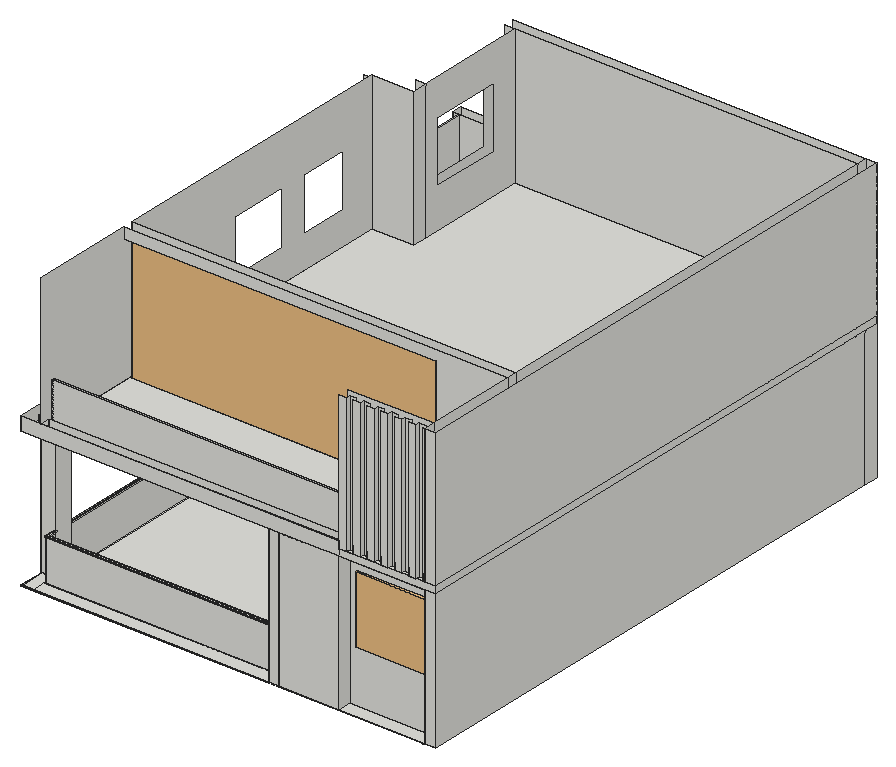
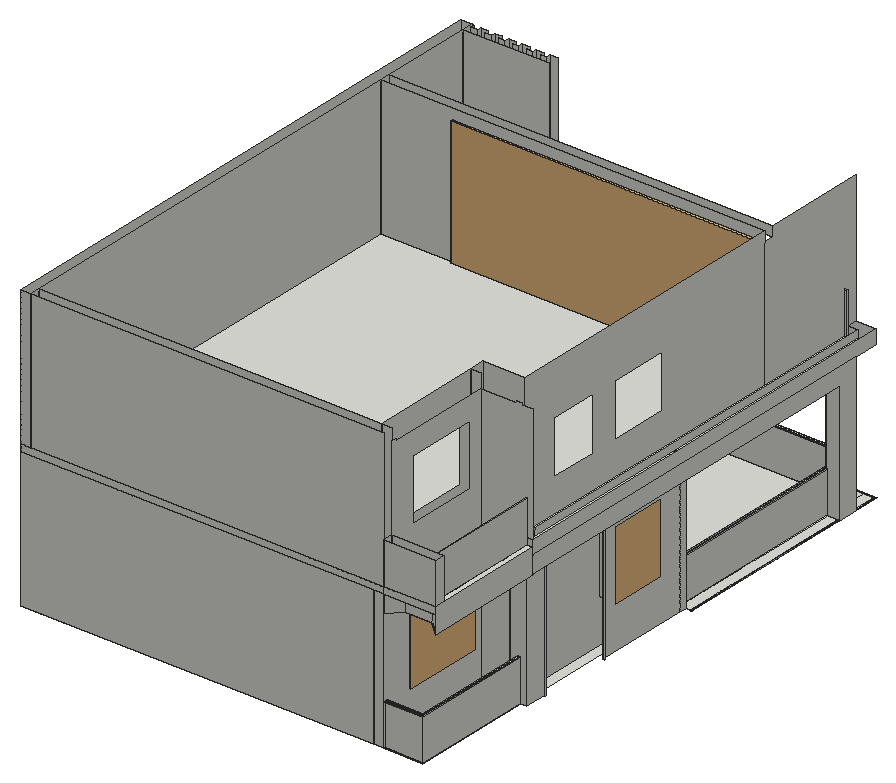
# SketchUp Ruby script. Lengths in inches.
U = 1.inch
M = Sketchup.active_model
def pt(a) = Geom::Point3d.new(a.map { |v| v * U })
def face(e, loops, mat)
  f = e.add_face(loops[0].map { |a| pt(a) })
  loops[1..].each { |l| e.add_face(l.map { |a| pt(a) }).erase! }
  f.material = f.back_material = mat if mat
  f
end
# faces: each face lists its corners as indices into pts; further lists are holes
def faces(e, pts, list, mat = nil) = list.each { |f| face(e, (f[0].is_a?(Array) ? f : [f]).map { |l| l.map { |i| pts[i] } }, mat) }
# xy, xz, yz: faces in a plane at the given z, y or x. An outline is a flat list of corners, or four numbers for a rectangle; further outlines are holes
def ring(l) = l.size == 4 ? [[l[0], l[1]], [l[2], l[1]], [l[2], l[3]], [l[0], l[3]]] : l.each_slice(2).to_a
def flat(e, list, mat, &to3) = list.each { |f| face(e, (f[0].is_a?(Array) ? f : [f]).map { |l| ring(l).map { |u, v| to3.(u, v) } }, mat) }
def xy(e, z, list, mat = nil) = flat(e, list, mat) { |x, y| [x, y, z] }
def xz(e, y, list, mat = nil) = flat(e, list, mat) { |x, z| [x, y, z] }
def yz(e, x, list, mat = nil) = flat(e, list, mat) { |y, z| [x, y, z] }
def lines(e, pts, list) = list.each { |a, b| e.add_line(pt(pts[a]), pt(pts[b])) }
# prism: a flat outline (further loops are holes) pulled along v
def prism(e, loops, v, mat = nil)
  f = face(e, loops, mat); d = Geom::Vector3d.new(v.map { |x| x * U })
  f.pushpull(f.normal.samedirection?(d) ? d.length : -d.length)
end
def box(e, o, s, mat = nil) = prism(e, [[o, [o[0] + s[0], o[1], o[2]], [o[0] + s[0], o[1] + s[1], o[2]], [o[0], o[1] + s[1], o[2]]]], [0, 0, s[2]], mat)
def at(x, y, z, deg = 0) = Geom::Transformation.translation(pt([x, y, z])) * Geom::Transformation.rotation(ORIGIN, Z_AXIS, deg.degrees)
def axes(o, x, y, z) = Geom::Transformation.new([*x, 0, *y, 0, *z, 0, *pt(o).to_a, 1])
def part(name) = M.definitions.add(name)
# library, detail: a bought-in or finely detailed component or shape, given as its bounding box
def library(name, o, s) = part(name).tap { |d| box(d.entities, o, s) }
def detail(e, o, s) = box(e.add_group.entities, o, s)
def put(e, d, t, mat = nil) = e.add_instance(d, t).tap { |i| i.material = mat if mat }
def group(e, t, mat = nil) = e.add_group.tap { |g| g.transformation = t; g.material = mat if mat }.entities
root = M.entities
c1 = library("Window 46-47",[-61.02,-2.17,0],[122.04,4.34,74.02])
c2 = library("Curtains 004",[-15.59,-2.26,0],[31.18,4.52,116.91])
c3 = library("Window 46-08",[-34.875,-3.16,0],[69.74,4.26,70.87])
c4 = library("Window 109 007",[-23.3125,-2.36,0.15],[46.625,4.71,46.28])
xy(root,383.75,[[17.25,9.625,17.25,210.85,17.3125,210.85,17.3125,9.6875,369.25,9.6875,369.25,9.625]])
xy(root,383.8125,[[17.125,9.5,17.125,210.85,17.25,210.85,17.25,9.625,369.25,9.625,369.25,9.5]])
xy(root,384,[[17.125,9.5,369.25,9.5,369.25,9.625,17.25,9.625,17.25,32.65,17.125,32.65],[17.25,9.625,369.25,9.625,369.25,9.6875,17.3125,9.6875,17.3125,32.65,17.25,32.65],[17.3125,9.6875,369.25,10.375],[17.3125,10.375,18.25,32.65],[18.25,10.375,27.25,32.65],
  [27.25,10.375,232.625,22.375],[232.625,10.375,241.625,210.85],[241.625,10.375,294.24,22.375],[294.24,10.375,369.25,22.375],[369.25,10.375,378.25,478.375],
  [27.25,22.375,232.625,22.375,232.625,23.46,28.34,23.46,28.34,32.65,27.25,32.65],[241.625,22.375,294.24,22.375,294.24,31.375,369.25,31.375,369.25,478.375,70.4375,478.375,70.4375,368.25,36.25,368.25,36.25,216.85,241.625,216.85],[294.24,22.375,369.25,31.375],[28.34,23.46,28.34,32.65,29.41,32.65,29.41,24.86,232.625,24.86,232.625,23.46],[29.41,24.86,231.54,24.86,231.54,25.95,232.625,25.95,232.625,210.85,193.58,210.85,193.58,216.85,77.58,216.85,77.58,210.85,30.5,210.85,30.5,49.65,29.41,49.65],
  [231.54,24.86,232.625,25.95],[16.4375,32.65,17.125,49.65],[17.125,32.65,17.25,49.65],[17.25,32.65,17.3125,49.65],[17.3125,32.65,29.41,49.65],
  [17.125,49.65,17.25,210.85],[17.25,49.65,17.3125,210.85],[17.3125,49.65,18.25,117.47],[18.25,49.65,27.25,210.85],[27.25,49.65,28.34,210.85],
  [28.34,49.65,29.41,210.85],[29.41,49.65,30.5,208.36],[17.3125,117.47,18.25,210.85],[29.41,208.36,30.5,209.76],[29.41,209.76,30.5,210.85],
  [22.125,210.85,27.25,216.85],[27.25,210.85,36.25,216.85],[36.25,210.85,77.58,216.85],[193.58,210.85,241.625,216.85],[27.25,216.85,36.25,384.4375],
  [36.25,368.25,70.4375,384.4375],[27.25,384.4375,28.1875,384.4375,28.1875,489.4375,61.84,489.4375,61.84,490.375,27.25,490.375],[28.1875,384.4375,28.1875,489.4375,61.84,489.4375,61.84,488.32,29.31,488.32,29.31,384.4375],[29.31,384.4375,30.25,384.4375,30.25,487.38,61.84,487.38,61.84,488.32,29.31,488.32],[30.25,384.4375,61.84,487.38],
  [61.84,384.4375,70.4375,490.375],[70.4375,478.375,378.25,490.375]])
xy(root,420,[[27.87,22.99,27.87,33.12,29.88,33.12,29.88,25.33,233.09,25.33,233.09,22.99],[27.57,23.02,27.57,30.81,27.87,31.1,27.87,23.02],[29.88,25.33,29.88,31.1,30.18,30.81,30.18,25.33],[27.79,49.1,29.96,211.4],[27.63,383.88,27.63,489.99,62.39,489.99,62.39,487.76,29.86,487.76,29.86,383.88]])
xy(root,420.5625,[[27.87,22.99,233.09,22.99,233.09,25.33,30.18,25.33,30.18,30.81,29.88,31.1,29.88,33.12,27.87,33.12,27.87,31.1,27.57,30.81,27.57,23.02,27.87,23.02],[27.63,383.88,29.86,383.88,29.86,487.76,62.39,487.76,62.39,489.99,27.63,489.99]])
xy(root,420.625,[[27.79,49.1,29.96,211.4]])
xy(root,422.29,[[22.125,240.52,36.25,287.64]])
xy(root,423.43,[[61.84,392.625,70.4375,463.11]])
xy(root,430.95,[[301.05,22.375,364.93,31.375]])
xy(root,478.55,[[61.84,392.625,70.4375,463.11]])
xy(root,479.79,[[22.125,240.52,36.25,287.64]])
xy(root,488.3125,[[16.4375,384.4375,16.4375,490.375,28.66,478.68,52.85,478.68,61.84,490.375,61.84,469.28,24.02,469.28,24.02,384.4375],[27.9,384.4375,61.84,465.4]])
xy(root,488.5,[[77.58,210.85,193.58,216.85]])
xy(root,488.88,[[16.4375,49.65,16.4375,384.4375,20.6875,384.4375,20.6875,365.41,29.41,365.41,29.41,49.65],[20.6875,365.41,22.125,384.4375]])
xy(root,489.89,[[301.05,22.375,364.93,31.375]])
xy(root,490.25,[[24.02,384.4375,24.02,469.28,61.84,469.28,61.84,465.4,27.9,465.4,27.9,384.4375]])
xy(root,504,[[[16.4375,10.375,16.4375,32.65,29.41,32.65,29.41,210.85,232.625,210.85,232.625,10.375],[52.17,29.78,206.86,176.97]],[232.625,10.375,241.625,210.85],[241.625,10.375,294.24,22.375],[294.24,10.375,369.25,22.375],[369.25,10.375,378.25,478.375],
  [241.625,22.375,241.625,216.85,70.4375,216.85,70.4375,478.375,369.25,478.375,369.25,31.375,294.24,31.375,294.24,22.375],[294.24,22.375,369.25,31.375],[294.24,22.375,369.25,31.375],[16.4375,32.65,29.41,210.85],[56.64,34.24,202.39,172.5],
  [16.4375,210.85,22.125,216.85],[22.125,210.85,29.41,216.85],[29.41,210.85,36.25,216.85],[36.25,210.85,61.84,216.85],[61.84,210.85,70.4375,216.85],
  [70.4375,210.85,241.625,216.85],[16.4375,216.85,22.125,216.85,22.125,300.74,20.6875,300.74,20.6875,384.4375,16.4375,384.4375],[22.125,216.85,22.125,300.74,20.6875,300.74,20.6875,384.4375,22.125,384.4375,22.125,365.41,29.41,365.41,29.41,216.85],[29.41,216.85,36.25,216.85,36.25,368.25,22.125,368.25,22.125,365.41,29.41,365.41],[36.25,216.85,61.84,368.25],
  [61.84,216.85,70.4375,368.25],[22.125,368.25,36.25,384.4375],[36.25,368.25,61.84,384.4375],[61.84,368.25,70.4375,384.4375],[61.84,384.4375,70.4375,490.375],
  [70.4375,478.375,378.25,490.375],[28.66,478.68,16.4375,490.375,61.84,490.375,52.85,478.68]])
xy(root,505.625,[[[52.17,29.78,206.86,176.97],[56.64,34.24,202.39,172.5]]])
xy(root,510,[[294.24,10.375,294.24,19.375,369.25,19.375,369.25,10.375,366.99,10.375,366.99,13.75,361.25,13.75,361.25,10.375,354.87,10.375,354.87,13.75,349.12,13.75,349.12,10.375,342.74,10.375,342.74,13.75,337,13.75,337,10.375,330.62,10.375,330.62,13.75,324.87,13.75,324.87,10.375,318.49,10.375,318.49,13.75,312.75,13.75,312.75,10.375,306.37,10.375,306.37,13.75,300.62,13.75,300.62,10.375],[300.62,10.375,306.37,13.75],[312.75,10.375,318.49,13.75],[324.87,10.375,330.62,13.75],[337,10.375,342.74,13.75],
  [349.12,10.375,354.87,13.75],[361.25,10.375,366.99,13.75],[369.25,10.375,378.25,490.375],[25.4375,19.375,25.4375,370.6,34.4375,370.6,34.4375,22.875,32.375,22.875,32.375,21.125,34.4375,21.125,34.4375,19.375],[294.24,19.375,369.25,19.375,369.25,100.375,306.375,100.375,306.375,109.375,34.4375,109.375,34.4375,24.625,294.24,24.625],
  [34.4375,19.375,294.24,19.375,294.24,24.625,34.4375,24.625,34.4375,22.875,292.49,22.875,292.49,21.125,34.4375,21.125],[32.375,21.125,34.4375,22.875],[34.4375,21.125,36.1875,22.875],[36.1875,21.125,292.49,22.875],[306.375,100.375,369.25,109.375],
  [34.4375,109.375,369.25,109.375,369.25,481.375,70.6875,481.375,70.6875,370.6,34.4375,370.6],[25.4375,370.6,70.6875,384.4375],[16.4375,384.4375,20.9375,481.375],[20.9375,384.4375,21.68,384.4375,21.68,480.63,22.63,480.63,22.63,384.4375,23.375,384.4375,23.375,481.375,20.9375,481.375],[21.68,384.4375,22.63,480.63],
  [23.375,384.4375,61.6875,481.375],[61.6875,384.4375,70.6875,481.375],[16.4375,481.375,61.84,490.375],[61.84,481.375,369.25,490.375]])
xz(root,9.5,[[17.125,383.8125,369.25,384]])
xz(root,9.625,[[17.25,383.75,369.25,383.8125],[17.25,383.8125,369.25,384]])
xz(root,9.6875,[[17.3125,383.75,369.25,384]])
xz(root,10.375,[[232.625,384,241.625,504],[241.625,384,294.24,504],[369.25,384,378.25,504],[16.4375,504,294.24,516],[294.24,504,378.25,510],
  [294.24,510,300.62,630],[306.37,510,312.75,630],[318.49,510,324.87,630],[330.62,510,337,630],[342.74,510,349.12,630],
  [354.87,510,361.25,630],[366.99,510,369.25,630],[369.25,510,378.25,630]])
xz(root,13.75,[[300.62,510,306.37,630],[312.75,510,318.49,630],[324.87,510,330.62,630],[337,510,342.74,630],[349.12,510,354.87,630],
  [361.25,510,366.99,630]])
xz(root,19.375,[[25.4375,510,34.4375,516],[34.4375,510,294.24,516],[294.24,510,369.25,630]])
xz(root,21.125,[[32.375,510,36.1875,546],[36.1875,510,292.49,546]])
xz(root,22.375,[[241.625,384,294.24,504],[[294.24,384,369.25,504],[301.05,430.95,364.93,489.89]]])
xz(root,22.875,[[32.375,510,36.1875,546],[36.1875,510,292.49,546]])
xz(root,22.99,[[27.87,420,233.09,420.5625]])
xz(root,23.02,[[27.57,420,27.87,420.5625],[27.87,420,231.54,420.5625]])
xz(root,23.46,[[28.34,384,232.625,420]])
xz(root,24.86,[[29.41,384,231.54,420],[231.54,384,232.625,420]])
xz(root,25.3,[[30.18,420,230.78,420.5625]])
xz(root,25.33,[[29.88,420,30.18,420.5625],[30.18,420,231.54,420.5625],[231.54,420,232.625,420.5625],[232.625,420,233.09,420.5625]])
xz(root,29.78,[[52.17,504,206.86,505.625]])
xz(root,31.375,[[[294.24,384,369.25,504],[301.05,430.95,364.93,489.89]]])
xz(root,32.65,[[16.4375,384,28.34,384,28.34,420,29.41,420,29.41,504,16.4375,504],[28.34,384,29.41,420]])
xz(root,33.12,[[27.87,420,29.88,420.5625]])
xz(root,34.24,[[56.64,504,202.39,505.625]])
xz(root,49.1,[[27.79,420,29.96,420.625]])
xz(root,49.65,[[16.4375,384,16.4375,488.88,29.41,488.88,29.41,420,28.34,420,28.34,384],[28.34,384,29.41,420]])
xz(root,100.375,[[306.375,510,369.25,510,369.25,630,34.4375,630,34.4375,621.1875,306.375,621.1875]])
xz(root,109.375,[[306.375,510,306.375,621.1875,34.4375,621.1875,34.4375,630,369.25,630,369.25,510]])
xz(root,172.5,[[56.64,504,202.39,505.625]])
xz(root,176.97,[[52.17,504,206.86,505.625]])
xz(root,210.85,[[17.25,383.75,17.3125,384],[17.125,383.8125,17.25,384],[22.125,384,28.34,384,28.34,420,27.79,420,27.79,420.625,29.91,420.625,29.91,420,29.41,420,29.41,384,77.58,384,77.58,488.5,193.58,488.5,193.58,384,232.625,384,232.625,504,22.125,504],[28.34,384,29.41,420],[232.625,384,241.625,504]])
xz(root,211.4,[[27.79,420,29.96,420.625]])
xz(root,216.85,[[22.125,384,36.25,504],[36.25,384,36.25,504,241.625,504,241.625,384,193.58,384,193.58,488.5,77.58,488.5,77.58,384]])
xz(root,240.52,[[22.125,422.29,36.25,479.79]])
xz(root,287.64,[[22.125,422.29,36.25,479.79]])
xz(root,300.74,[[20.6875,384,22.125,504]])
xz(root,365.41,[[20.6875,384,22.125,488.88],[22.125,488.88,29.41,504]])
xz(root,368.25,[[36.25,384,70.4375,504]])
xz(root,370.6,[[34.4375,510,70.6875,630]])
xz(root,383.88,[[27.63,420,29.86,420.5625]])
xz(root,384.4375,[[22.125,384,22.125,488.3125,24.02,488.3125,24.02,490.25,27.9,490.25,27.9,488.3125,36.25,488.3125,36.25,384,29.31,384,29.31,420,28.1875,420,28.1875,384],[36.25,384,61.84,488.3125],[61.84,384,70.4375,504],[16.4375,488.3125,20.6875,488.88],[20.6875,488.3125,22.125,488.88],
  [22.125,488.3125,22.125,504,36.25,504,36.25,488.3125,27.9,488.3125,27.9,490.25,24.02,490.25,24.02,488.3125],[36.25,488.3125,61.84,504],[16.4375,488.88,20.6875,504],[20.6875,488.88,22.125,504],[16.4375,510,21.68,516],
  [25.4375,510,25.4375,516,22.63,516,22.63,546,23.07,546,23.07,546.75,20.82,546.75,20.82,546,21.68,546,21.68,516,16.4375,516,16.4375,618.0625,26.0625,618.0625,26.0625,619.6875,30.13,619.6875,30.13,618.0625,61.6875,618.0625,61.6875,510],[21.68,510,22.63,516],[22.63,510,25.4375,516],[61.6875,510,70.6875,630]])
xz(root,392.625,[[61.84,423.43,70.4375,478.55]])
xz(root,463.11,[[61.84,423.43,70.4375,478.55]])
xz(root,465.4,[[27.9,488.3125,61.84,490.25]])
xz(root,469.28,[[24.02,488.3125,61.84,490.25]])
xz(root,478.375,[[70.4375,384,369.25,504],[369.25,384,378.25,504]])
xz(root,478.68,[[28.66,488.3125,52.85,504]])
xz(root,480.63,[[21.68,510,22.63,546]])
xz(root,481.375,[[16.4375,510,61.6875,546],[61.6875,510,61.84,546],[61.84,510,70.6875,630],[70.6875,510,369.25,630]])
xz(root,487.76,[[29.86,420,58.84,420.5625],[58.84,420,62.39,420.5625]])
xz(root,487.93,[[29.7,420,60.33,420.5625]])
xz(root,488.32,[[29.31,384,58.84,420],[58.84,384,61.84,420]])
xz(root,489.4375,[[28.1875,384,61.84,420]])
xz(root,489.83,[[27.8,420,60.33,420.5625]])
xz(root,489.99,[[27.63,420,61.84,420.5625],[61.84,420,62.39,420.5625]])
xz(root,490.375,[[61.84,384,70.4375,504],[70.4375,384,378.25,504],[16.4375,504,61.84,510],[61.84,504,378.25,510],[16.4375,510,61.84,546],
  [61.84,510,369.25,630],[369.25,510,378.25,630]])
yz(root,16.4375,[[32.65,384,32.65,504,384.4375,504,384.4375,488.88,49.65,488.88,49.65,384],[384.4375,488.3125,490.375,510],[10.375,504,384.4375,516],[481.375,510,490.375,546]])
yz(root,17.125,[[9.5,383.8125,10.375,384],[10.375,383.8125,32.65,384],[32.65,383.8125,49.65,384],[49.65,383.8125,117.47,384],[117.47,383.8125,210.85,384]])
yz(root,17.25,[[9.625,383.75,10.375,383.8125],[10.375,383.75,32.65,383.8125],[32.65,383.75,49.65,383.8125],[49.65,383.75,117.47,383.8125],[117.47,383.75,210.85,383.8125],
  [9.625,383.8125,10.375,384],[10.375,383.8125,32.65,384],[32.65,383.8125,49.65,384],[49.65,383.8125,117.47,384],[117.47,383.8125,210.85,384]])
yz(root,17.3125,[[9.6875,383.75,10.375,384],[10.375,383.75,32.65,384],[32.65,383.75,49.65,384],[49.65,383.75,117.47,384],[117.47,383.75,210.85,384]])
yz(root,21.68,[[384.4375,510,480.63,546]])
yz(root,22.125,[[210.85,384,216.85,504],[[216.85,384,300.74,504],[240.52,422.29,287.64,479.79]],[365.41,384,384.4375,488.88],[365.41,488.88,384.4375,504]])
yz(root,22.63,[[384.4375,510,480.63,546]])
yz(root,24.02,[[384.4375,488.3125,469.28,490.25]])
yz(root,25.4375,[[19.375,510,370.6,516],[370.6,510,384.4375,516]])
yz(root,27.57,[[23.02,420,30.81,420.5625]])
yz(root,27.63,[[383.88,420,489.99,420.5625]])
yz(root,27.79,[[49.1,420,210.85,420.625],[210.85,420,211.4,420.625]])
yz(root,27.8,[[385.95,420,489.83,420.5625]])
yz(root,27.84,[[51.23,420,209.76,420.625]])
yz(root,27.87,[[22.99,420,23.02,420.5625],[23.02,420,31.1,420.5625],[31.1,420,33.12,420.5625]])
yz(root,27.9,[[384.4375,488.3125,465.4,490.25]])
yz(root,28.1875,[[384.4375,384,489.4375,420]])
yz(root,28.34,[[23.46,384,32.65,420],[49.65,384,210.85,420]])
yz(root,29.31,[[384.4375,384,387.43,420],[387.43,384,488.32,420]])
yz(root,29.41,[[24.86,384,32.65,420],[32.65,384,49.65,384,49.65,488.88,365.41,488.88,365.41,504,32.65,504],[49.65,384,208.36,420],[208.36,384,209.76,420],[209.76,384,210.85,420]])
yz(root,29.7,[[385.95,420,487.93,420.5625]])
yz(root,29.86,[[383.88,420,387.43,420.5625],[387.43,420,487.76,420.5625]])
yz(root,29.88,[[25.33,420,31.1,420.5625],[31.1,420,33.12,420.5625]])
yz(root,29.91,[[51.23,420,209.27,420.625]])
yz(root,29.96,[[49.1,420,208.36,420.625],[208.36,420,209.76,420.625],[209.76,420,211.4,420.625]])
yz(root,30.18,[[25.3,420,25.33,420.5625],[25.33,420,30.81,420.5625]])
yz(root,32.375,[[21.125,510,22.875,546]])
yz(root,34.4375,[[[19.375,510,109.375,510,109.375,621.1875,100.375,621.1875,100.375,630,10.375,630,10.375,516,19.375,516],[20.75,546,23.0625,546.5625]],[[109.375,510,370.6,630],[221.19,538.43,272.76,584.75],[297.07,538.43,339.01,584.75]]])
yz(root,36.25,[[[216.85,384,368.25,504],[240.52,422.29,287.64,479.79]],[368.25,384,384.4375,504]])
yz(root,52.17,[[29.78,504,176.97,505.625]])
yz(root,56.64,[[34.24,504,172.5,505.625]])
yz(root,61.6875,[[[384.4375,510,384.4375,618.0625,477.3,618.0625,477.3,619.6875,481.375,619.6875,481.375,510],[396.46,544.6,458.58,598.04]]])
yz(root,61.84,[[[384.4375,384,384.4375,488.3125,465.4,488.3125,465.4,490.25,469.28,490.25,469.28,488.3125,490.375,488.3125,490.375,384,489.4375,384,489.4375,420,489.99,420,489.99,420.5625,487.93,420.5625,487.93,420,488.32,420,488.32,384],[392.625,423.43,463.11,478.55]],[488.32,384,489.4375,420],[384.4375,488.3125,384.4375,504,490.375,504,490.375,488.3125,469.28,488.3125,469.28,490.25,465.4,490.25,465.4,488.3125],[481.375,510,490.375,546]])
yz(root,62.39,[[487.76,420,489.99,420.5625]])
yz(root,70.4375,[[368.25,384,384.4375,504],[[384.4375,384,478.375,504],[392.625,423.43,463.11,478.55]],[478.375,384,490.375,504]])
yz(root,70.6875,[[370.6,510,384.4375,630],[[384.4375,510,481.375,630],[396.46,544.6,458.58,598.04]]])
yz(root,77.58,[[210.85,384,216.85,488.5]])
yz(root,193.58,[[210.85,384,216.85,488.5]])
yz(root,202.39,[[34.24,504,172.5,505.625]])
yz(root,206.86,[[29.78,504,176.97,505.625]])
yz(root,232.625,[[10.375,384,10.375,504,210.85,504,210.85,384,24.86,384,24.86,420,25.33,420,25.33,420.5625,23.02,420.5625,23.02,420,23.46,420,23.46,384],[23.46,384,24.86,420]])
yz(root,233.09,[[22.99,420,25.33,420.5625]])
yz(root,241.625,[[10.375,384,22.375,504],[22.375,384,210.85,504],[210.85,384,216.85,504]])
yz(root,292.49,[[21.125,510,22.875,546]])
yz(root,294.24,[[10.375,384,22.375,504],[22.375,384,31.375,504],[10.375,510,19.375,516]])
yz(root,300.62,[[10.375,510,13.75,630]])
yz(root,301.05,[[22.375,430.95,31.375,489.89]])
yz(root,306.37,[[10.375,510,13.75,516]])
yz(root,306.375,[[100.375,510,109.375,621.1875]])
yz(root,312.75,[[10.375,510,13.75,630]])
yz(root,318.49,[[10.375,510,13.75,516]])
yz(root,324.87,[[10.375,510,13.75,630]])
yz(root,330.62,[[10.375,510,13.75,516]])
yz(root,337,[[10.375,510,13.75,630]])
yz(root,342.74,[[10.375,510,13.75,516]])
yz(root,349.12,[[10.375,510,13.75,630]])
yz(root,354.87,[[10.375,510,13.75,516]])
yz(root,361.25,[[10.375,510,13.75,630]])
yz(root,364.93,[[22.375,430.95,31.375,489.89]])
yz(root,366.99,[[10.375,510,13.75,516]])
yz(root,369.25,[[9.625,383.75,9.6875,384],[9.5,383.8125,9.625,384],[10.375,384,22.375,504],[22.375,384,31.375,504],[31.375,384,478.375,504],
  [10.375,510,19.375,630],[19.375,510,100.375,630],[100.375,510,109.375,630],[109.375,510,481.375,630],[481.375,510,490.375,630]])
yz(root,378.25,[[10.375,384,478.375,504],[478.375,384,490.375,504],[10.375,504,490.375,510],[10.375,510,490.375,630]])
p = [[27.57,30.81,420.5625],[27.87,31.1,420.5625],[27.87,31.1,420],[27.57,30.81,420],[29.88,31.1,420.5625],[30.18,30.81,420.5625],
  [30.18,30.81,420],[29.88,31.1,420],[16.4375,490.375,504],[28.66,478.68,504],[28.66,478.68,488.3125],[16.4375,490.375,488.3125],
  [52.85,478.68,504],[61.84,490.375,504],[61.84,490.375,488.3125],[52.85,478.68,488.3125],[30.5,25.95,384],[229.05,25.95,384],
  [30.5,32.65,384],[29.41,32.65,384]]
faces(root,p,[[0,1,2,3],[4,5,6,7],[8,9,10,11],[12,13,14,15]])
lines(root,p,[[16,17],[18,16],[18,19]])
put(root,c1,axes([135.58,216.85,384],[1,0,0],[0,1,0],[0,0,1.41185]))
put(root,c2,at(353.66,33.63,387.09))
put(root,c2,at(181.9375,219.1,387.09))
put(root,c2,at(85.9375,219.1,387.09))
put(root,c2,at(72.7,401.71,387.09,90))
put(root,c2,at(72.7,453.47,387.09,90))
put(root,c3,axes([65.67,427.87,418.55],[0,1.01061,0],[1.76,0,0],[0,0,0.84667]))
put(root,c3,axes([22.64,263.82,421.61],[0,0.68821,0],[-1,0,0],[0,0,0.84667]))
put(root,c4,axes([332.94,22.375,430.91],[1.36801,0,0],[0,1,0],[0,0,1.27025]))
put(root,c1,axes([171.1,109.375,510],[2.21675,0,0],[0,1,0],[0,0,1.5022]))
